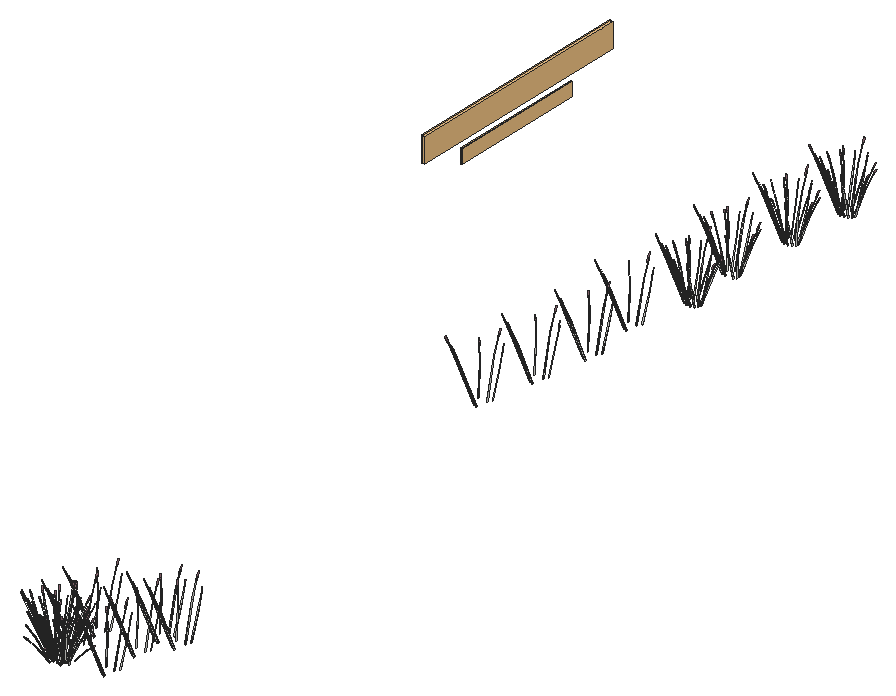
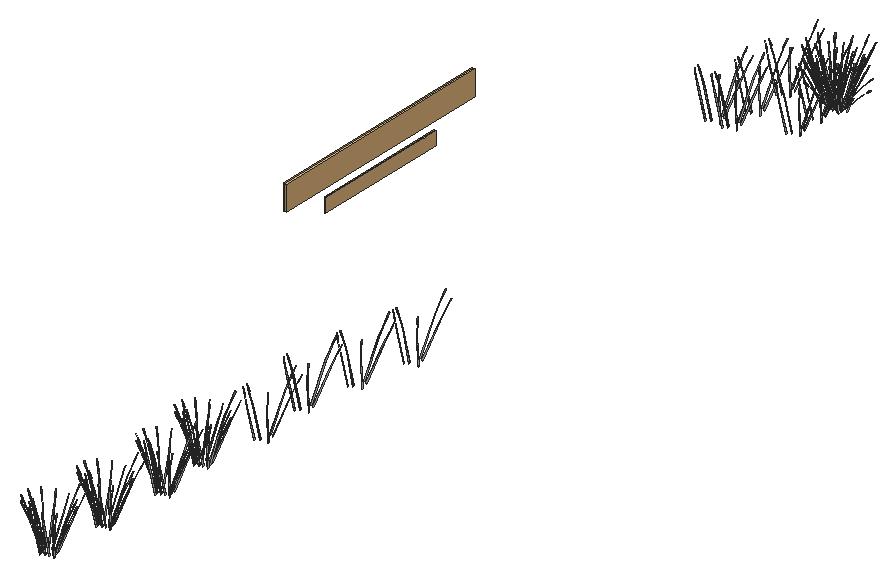
# SketchUp Ruby script. Lengths in inches.
U = 1.inch
M = Sketchup.active_model
def pt(a) = Geom::Point3d.new(a.map { |v| v * U })
def face(e, loops, mat)
  f = e.add_face(loops[0].map { |a| pt(a) })
  loops[1..].each { |l| e.add_face(l.map { |a| pt(a) }).erase! }
  f.material = f.back_material = mat if mat
  f
end
# faces: each face lists its corners as indices into pts; further lists are holes
def faces(e, pts, list, mat = nil) = list.each { |f| face(e, (f[0].is_a?(Array) ? f : [f]).map { |l| l.map { |i| pts[i] } }, mat) }
# xy, xz, yz: faces in a plane at the given z, y or x. An outline is a flat list of corners, or four numbers for a rectangle; further outlines are holes
def ring(l) = l.size == 4 ? [[l[0], l[1]], [l[2], l[1]], [l[2], l[3]], [l[0], l[3]]] : l.each_slice(2).to_a
def flat(e, list, mat, &to3) = list.each { |f| face(e, (f[0].is_a?(Array) ? f : [f]).map { |l| ring(l).map { |u, v| to3.(u, v) } }, mat) }
def xy(e, z, list, mat = nil) = flat(e, list, mat) { |x, y| [x, y, z] }
def xz(e, y, list, mat = nil) = flat(e, list, mat) { |x, z| [x, y, z] }
def yz(e, x, list, mat = nil) = flat(e, list, mat) { |y, z| [x, y, z] }
def lines(e, pts, list) = list.each { |a, b| e.add_line(pt(pts[a]), pt(pts[b])) }
# prism: a flat outline (further loops are holes) pulled along v
def prism(e, loops, v, mat = nil)
  f = face(e, loops, mat); d = Geom::Vector3d.new(v.map { |x| x * U })
  f.pushpull(f.normal.samedirection?(d) ? d.length : -d.length)
end
def box(e, o, s, mat = nil) = prism(e, [[o, [o[0] + s[0], o[1], o[2]], [o[0] + s[0], o[1] + s[1], o[2]], [o[0], o[1] + s[1], o[2]]]], [0, 0, s[2]], mat)
def at(x, y, z, deg = 0) = Geom::Transformation.translation(pt([x, y, z])) * Geom::Transformation.rotation(ORIGIN, Z_AXIS, deg.degrees)
def axes(o, x, y, z) = Geom::Transformation.new([*x, 0, *y, 0, *z, 0, *pt(o).to_a, 1])
def part(name) = M.definitions.add(name)
# library, detail: a bought-in or finely detailed component or shape, given as its bounding box
def library(name, o, s) = part(name).tap { |d| box(d.entities, o, s) }
def detail(e, o, s) = box(e.add_group.entities, o, s)
def put(e, d, t, mat = nil) = e.add_instance(d, t).tap { |i| i.material = mat if mat }
def group(e, t, mat = nil) = e.add_group.tap { |g| g.transformation = t; g.material = mat if mat }.entities
root = M.entities
M.materials.add("LightPink_Translucent").color = [144, 107, 117]
c1 = part("blade")
p = [[2.15,0.21,22],[0,0.17,0],[0.09,0.45,0],[2.18,0.31,22],[2.29,0.31,22],[0.38,0.45,0],
  [2.48,0.24,33],[2.49,0.24,33],[2.48,0.22,33]]
faces(c1.entities,p,[[0,1,2,3],[4,5,2,3],[6,3,4,7],[8,0,3,6]])
c2 = part("seeds")
p = [[0.3,-0.1,1.38],[-0.01,-0.03,1.59],[-0.01,-0.03,0.03],[0.14,-0.07,-0.07],[0.29,-0.03,3],[0.15,0.01,3.11]]
faces(c2.entities,p,[[0,1,2,3],[1,0,4,5]],"LightPink_Translucent")
c3 = part("blade with seeds")
put(c3.entities,c1,at(0,0,0))
put(c3.entities,c2,axes([2.4,0.25,30.99],[1.5799,-0.05474,1.17369],[-0.12525,1.92788,0.29478],[-0.07173,-0.02425,1.56792]))
c4 = library("WELLNESS CLUB",[0.17,0,0],[97.05,9.88,1])
c5 = library("MAXX AURA",[0.96,0,0],[68.67,9.71,1])
put(root,c3,axes([53.25,597.27,47.05],[-0.69728,-0.64842,0.35414],[0.79619,-0.61382,-0.4572],[0.40453,0.09339,0.87481]))
put(root,c3,axes([54.39,595.45,47.05],[-1.01846,-0.28891,0.35414],[0.29705,-0.84289,-0.4572],[0.41005,-0.07729,0.87481]))
put(root,c3,axes([45.72,592.11,47.05],[0.69728,0.64842,0.35414],[-0.79619,0.61382,-0.4572],[-0.40453,-0.09339,0.87481]))
put(root,c3,axes([46.18,597.63,47.05],[0.82919,-0.54528,0.35414],[0.78493,0.62262,-0.4572],[-0.11943,0.31634,0.87481]))
put(root,c3,axes([44.74,595.95,47.05],[1.06674,-0.14801,0.35414],[0.28168,0.84611,-0.4572],[-0.30569,0.22726,0.87481]))
put(root,c3,axes([51.09,598.4,47.05],[-0.18927,-0.83419,0.35414],[1.08199,-0.22027,-0.4572],[0.29062,0.23905,0.87481]))
put(root,c3,axes([54.22,593.43,47.05],[-1.06674,0.14801,0.35414],[-0.28168,-0.84611,-0.4572],[0.30569,-0.22726,0.87481]))
put(root,c3,axes([44.57,593.92,47.05],[1.01846,0.28891,0.35414],[-0.29705,0.84289,-0.4572],[-0.41005,0.07729,0.87481]))
put(root,c3,axes([52.78,591.74,47.05],[-0.82919,0.54528,0.35414],[-0.78493,-0.62262,-0.4572],[0.11943,-0.31634,0.87481]))
put(root,c3,axes([47.87,590.98,47.05],[0.18927,0.83419,0.35414],[-1.08199,0.22027,-0.4572],[-0.29062,-0.23905,0.87481]))
put(root,c3,axes([51.3,647.54,47.05],[0.36946,-0.79643,0.35414],[1.07787,0.23229,-0.4572],[0.09883,0.32066,0.87481]))
put(root,c3,axes([53.25,639.86,47.05],[-0.36946,0.79643,0.35414],[-1.07787,-0.23229,-0.4572],[-0.09883,-0.32066,0.87481]))
put(root,c3,axes([56.04,646.28,47.05],[-0.69728,-0.64842,0.35414],[0.79619,-0.61382,-0.4572],[0.40453,0.09339,0.87481]))
put(root,c3,axes([57.1875,644.46,47.05],[-1.01846,-0.28891,0.35414],[0.29705,-0.84289,-0.4572],[0.41005,-0.07729,0.87481]))
put(root,c3,axes([48.51,641.12,47.05],[0.69728,0.64842,0.35414],[-0.79619,0.61382,-0.4572],[-0.40453,-0.09339,0.87481]))
put(root,c3,axes([48.97,646.64,47.05],[0.82919,-0.54528,0.35414],[0.78493,0.62262,-0.4572],[-0.11943,0.31634,0.87481]))
put(root,c3,axes([47.53,644.96,47.05],[1.06674,-0.14801,0.35414],[0.28168,0.84611,-0.4572],[-0.30569,0.22726,0.87481]))
put(root,c3,axes([53.88,647.41,47.05],[-0.18927,-0.83419,0.35414],[1.08199,-0.22027,-0.4572],[0.29062,0.23905,0.87481]))
put(root,c3,axes([57.02,642.44,47.05],[-1.06674,0.14801,0.35414],[-0.28168,-0.84611,-0.4572],[0.30569,-0.22726,0.87481]))
put(root,c3,axes([47.36,642.93,47.05],[1.01846,0.28891,0.35414],[-0.29705,0.84289,-0.4572],[-0.41005,0.07729,0.87481]))
put(root,c3,axes([55.58,640.75,47.05],[-0.82919,0.54528,0.35414],[-0.78493,-0.62262,-0.4572],[0.11943,-0.31634,0.87481]))
put(root,c3,axes([50.66,639.99,47.05],[0.18927,0.83419,0.35414],[-1.08199,0.22027,-0.4572],[-0.29062,-0.23905,0.87481]))
put(root,c3,axes([55.84,691.87,47.05],[0.36946,-0.79643,0.35414],[1.07787,0.23229,-0.4572],[0.09883,0.32066,0.87481]))
put(root,c3,axes([57.79,684.1875,47.05],[-0.36946,0.79643,0.35414],[-1.07787,-0.23229,-0.4572],[-0.09883,-0.32066,0.87481]))
put(root,c3,axes([60.58,690.61,47.05],[-0.69728,-0.64842,0.35414],[0.79619,-0.61382,-0.4572],[0.40453,0.09339,0.87481]))
put(root,c3,axes([61.73,688.79,47.05],[-1.01846,-0.28891,0.35414],[0.29705,-0.84289,-0.4572],[0.41005,-0.07729,0.87481]))
put(root,c3,axes([53.05,685.44,47.05],[0.69728,0.64842,0.35414],[-0.79619,0.61382,-0.4572],[-0.40453,-0.09339,0.87481]))
put(root,c3,axes([53.51,690.97,47.05],[0.82919,-0.54528,0.35414],[0.78493,0.62262,-0.4572],[-0.11943,0.31634,0.87481]))
put(root,c3,axes([52.07,689.29,47.05],[1.06674,-0.14801,0.35414],[0.28168,0.84611,-0.4572],[-0.30569,0.22726,0.87481]))
put(root,c3,axes([58.42,691.74,47.05],[-0.18927,-0.83419,0.35414],[1.08199,-0.22027,-0.4572],[0.29062,0.23905,0.87481]))
put(root,c3,axes([61.56,686.77,47.05],[-1.06674,0.14801,0.35414],[-0.28168,-0.84611,-0.4572],[0.30569,-0.22726,0.87481]))
put(root,c3,axes([51.9,687.26,47.05],[1.01846,0.28891,0.35414],[-0.29705,0.84289,-0.4572],[-0.41005,0.07729,0.87481]))
put(root,c3,axes([60.12,685.08,47.05],[-0.82919,0.54528,0.35414],[-0.78493,-0.62262,-0.4572],[0.11943,-0.31634,0.87481]))
put(root,c3,axes([55.2,684.32,47.05],[0.18927,0.83419,0.35414],[-1.08199,0.22027,-0.4572],[-0.29062,-0.23905,0.87481]))
put(root,c3,axes([52.33,559.71,47.05],[0.36946,-0.79643,0.35414],[1.07787,0.23229,-0.4572],[0.09883,0.32066,0.87481]))
put(root,c3,axes([54.29,552.02,47.05],[-0.36946,0.79643,0.35414],[-1.07787,-0.23229,-0.4572],[-0.09883,-0.32066,0.87481]))
put(root,c3,axes([57.08,558.45,47.05],[-0.69728,-0.64842,0.35414],[0.79619,-0.61382,-0.4572],[0.40453,0.09339,0.87481]))
put(root,c3,axes([58.22,556.63,47.05],[-1.01846,-0.28891,0.35414],[0.29705,-0.84289,-0.4572],[0.41005,-0.07729,0.87481]))
put(root,c3,axes([49.55,553.28,47.05],[0.69728,0.64842,0.35414],[-0.79619,0.61382,-0.4572],[-0.40453,-0.09339,0.87481]))
put(root,c3,axes([50.01,558.81,47.05],[0.82919,-0.54528,0.35414],[0.78493,0.62262,-0.4572],[-0.11943,0.31634,0.87481]))
put(root,c3,axes([48.57,557.12,47.05],[1.06674,-0.14801,0.35414],[0.28168,0.84611,-0.4572],[-0.30569,0.22726,0.87481]))
put(root,c3,axes([54.92,559.57,47.05],[-0.18927,-0.83419,0.35414],[1.08199,-0.22027,-0.4572],[0.29062,0.23905,0.87481]))
put(root,c3,axes([58.05,554.6,47.05],[-1.06674,0.14801,0.35414],[-0.28168,-0.84611,-0.4572],[0.30569,-0.22726,0.87481]))
put(root,c3,axes([48.4,555.1,47.05],[1.01846,0.28891,0.35414],[-0.29705,0.84289,-0.4572],[-0.41005,0.07729,0.87481]))
put(root,c3,axes([56.61,552.92,47.05],[-0.82919,0.54528,0.35414],[-0.78493,-0.62262,-0.4572],[0.11943,-0.31634,0.87481]))
put(root,c3,axes([51.7,552.15,47.05],[0.18927,0.83419,0.35414],[-1.08199,0.22027,-0.4572],[-0.29062,-0.23905,0.87481]))
put(root,c3,axes([24.8,17.97,46.96],[0.09085,0.10335,1.77383],[-0.43798,0.92907,-0.16761],[-0.44357,0.00672,0.31391]))
put(root,c3,axes([28.63,15.28,46.96],[-0.02286,0.12414,1.77383],[-1.12758,0.45052,-0.16761],[-0.33182,-0.23029,0.31391]))
put(root,c3,axes([31.04,27.05,46.96],[0.00363,-0.12539,1.77383],[1.0502,-0.55319,-0.16761],[0.36479,0.19745,0.31391]))
put(root,c3,axes([21.63,23.06,46.96],[0.1564,0.02778,1.77383],[0.48382,0.91506,-0.16761],[-0.32016,0.24017,0.31391]))
put(root,c3,axes([38.57,20.74,46.96],[-0.16006,-0.00787,1.77383],[-0.66468,-0.8428,-0.16761],[0.26693,-0.27711,0.31391]))
put(root,c3,axes([38.28,26.01,46.96],[-0.11081,-0.09067,1.77383],[0.2424,-0.97188,-0.16761],[0.43649,-0.06209,0.31391]))
put(root,c3,axes([23.79,27.83,46.96],[0.13903,-0.06253,1.77383],[1.14912,0.41591,-0.16761],[-0.027,0.34629,0.31391]))
put(root,c3,axes([35.27,16.8,46.96],[-0.12446,0.07911,1.77383],[-1.21937,-0.26689,-0.16761],[-0.04414,-0.34521,0.31391]))
put(root,c3,axes([26.65,25.27,47.65],[1.34686,0.05131,-0.13498],[-0.03681,0.97156,-0.74919],[-0.09356,0.37418,1.13838]))
put(root,c3,axes([28.95,17.64,47.68],[-0.81789,0.99285,-0.13619],[-1.18445,-0.572,-0.75594],[-0.41173,-0.28051,1.14864]))
put(root,c3,axes([28.7,17.71,46.98],[0.55698,-0.6579,0.0643],[0.79316,0.38303,0.50621],[-0.25643,-0.21093,0.77189]))
put(root,c3,axes([29.17,26.74,46.98],[-0.90301,0.35198,0.0643],[-0.44199,-0.64184,0.50621],[0.08721,0.28293,0.77189]))
put(root,c3,axes([36.19,20.78,46.98],[0.8413,0.43556,0.0643],[-0.48981,0.62025,0.50621],[0.26973,-0.20053,0.77189]))
put(root,c3,axes([36.32,23.2,46.98],[0.4501,0.70615,0.0643],[-0.82077,0.34564,0.50621],[0.36181,-0.0682,0.77189]))
put(root,c3,axes([26.08,19,46.98],[0.06171,-0.78753,0.0643],[0.9318,0.02159,0.50621],[-0.35694,-0.08241,0.77189]))
put(root,c3,axes([34.54,18.73,46.98],[1.00708,0.04826,0.0643],[-0.02761,0.72867,0.50621],[0.10538,-0.27912,0.77189]))
put(root,c3,axes([34.88,25.34,46.98],[-0.06171,0.78753,0.0643],[-0.9318,-0.02159,0.50621],[0.35694,0.08241,0.77189]))
put(root,c3,axes([24.77,23.57,46.98],[-0.8413,-0.43556,0.0643],[0.48981,-0.62025,0.50621],[-0.26973,0.20053,0.77189]))
put(root,c3,axes([31.79,17.61,46.98],[0.90301,-0.35198,0.0643],[0.44199,0.64184,0.50621],[-0.08721,-0.28293,0.77189]))
put(root,c3,axes([24.65,21.15,46.98],[-0.4501,-0.70615,0.0643],[0.82077,-0.34564,0.50621],[-0.36181,0.0682,0.77189]))
put(root,c3,axes([32.26,26.64,46.98],[-0.55698,0.6579,0.0643],[-0.79316,-0.38303,0.50621],[0.25643,0.21093,0.77189]))
put(root,c3,axes([26.43,25.61,46.98],[-1.00708,-0.04826,0.0643],[0.02761,-0.72867,0.50621],[-0.10538,0.27912,0.77189]))
put(root,c3,axes([31.47,17.68,46.98],[1.20755,0.27075,0.48003],[-0.41292,0.89013,0.3958],[-0.07257,-0.35005,0.9933]))
put(root,c3,axes([34.97,25.09,46.98],[-0.90362,0.68241,0.48003],[-0.77932,-0.72471,0.3958],[0.42395,0.12588,0.9933]))
put(root,c3,axes([36.23,22.95,46.98],[-0.34623,0.9443,0.48003],[-1.13828,-0.3229,0.3958],[0.44763,-0.05675,0.9933]))
put(root,c3,axes([25.01,23.75,46.98],[-0.30393,-0.95317,0.48003],[1.19224,-0.16542,0.3958],[-0.35138,0.22417,0.9933]))
put(root,c3,axes([26.75,25.68,46.98],[-0.87265,-0.70663,0.48003],[0.92674,-0.60943,0.3958],[-0.16097,0.33153,0.9933]))
put(root,c3,axes([34.22,18.67,46.98],[0.87265,0.70663,0.48003],[-0.92674,0.60943,0.3958],[0.16097,-0.33153,0.9933]))
put(root,c3,axes([24.73,21.4,46.98],[0.34623,-0.9443,0.48003],[1.13828,0.3229,0.3958],[-0.44763,0.05675,0.9933]))
put(root,c3,axes([35.96,20.6,46.98],[0.30393,0.95317,0.48003],[-1.19224,0.16542,0.3958],[0.35138,-0.22417,0.9933]))
put(root,c3,axes([32.5,26.45,46.98],[-1.21888,0.23767,0.48003],[-0.21154,-0.93233,0.3958],[0.28666,0.27478,0.9933]))
put(root,c3,axes([31.04,42.73,47.0625],[-1.20755,-0.27075,0.53283],[0.41292,-0.89013,0.43934],[0.07257,0.35005,1.10256]))
put(root,c3,axes([30.74,61.76,47.0625],[-1.20755,-0.27075,0.53283],[0.41292,-0.89013,0.43934],[0.07257,0.35005,1.10256]))
put(root,c3,axes([62.51,30.73,47.0625],[-1.20755,-0.27075,0.53283],[0.41292,-0.89013,0.43934],[0.07257,0.35005,1.10256]))
put(root,c3,axes([62.3,58.02,47.0625],[-1.20755,-0.27075,0.53283],[0.41292,-0.89013,0.43934],[0.07257,0.35005,1.10256]))
put(root,c3,axes([62.3,78.73,47.0625],[-1.20755,-0.27075,0.53283],[0.41292,-0.89013,0.43934],[0.07257,0.35005,1.10256]))
put(root,c3,axes([74.3,78.73,47.0625],[-1.20755,-0.27075,0.53283],[0.41292,-0.89013,0.43934],[0.07257,0.35005,1.10256]))
put(root,c3,axes([33.46,397.47,47.0625],[-1.20755,-0.27075,0.53283],[0.41292,-0.89013,0.43934],[0.07257,0.35005,1.10256]))
put(root,c3,axes([41.61,437.16,47.0625],[-1.20755,-0.27075,0.53283],[0.41292,-0.89013,0.43934],[0.07257,0.35005,1.10256]))
put(root,c3,axes([47.97,476.43,47.0625],[-1.20755,-0.27075,0.53283],[0.41292,-0.89013,0.43934],[0.07257,0.35005,1.10256]))
put(root,c3,axes([44.35,516.68,47.0625],[-1.20755,-0.27075,0.53283],[0.41292,-0.89013,0.43934],[0.07257,0.35005,1.10256]))
put(root,c3,axes([48.49,599.18,47.0625],[-1.20755,-0.27075,0.53283],[0.41292,-0.89013,0.43934],[0.07257,0.35005,1.10256]))
put(root,c3,axes([51.28,648.19,47.0625],[-1.20755,-0.27075,0.53283],[0.41292,-0.89013,0.43934],[0.07257,0.35005,1.10256]))
put(root,c3,axes([55.82,692.52,47.0625],[-1.20755,-0.27075,0.53283],[0.41292,-0.89013,0.43934],[0.07257,0.35005,1.10256]))
put(root,c3,axes([52.32,560.36,47.0625],[-1.20755,-0.27075,0.53283],[0.41292,-0.89013,0.43934],[0.07257,0.35005,1.10256]))
put(root,c3,axes([27.17,35.07,47.09],[1.01205,-0.7643,0.53763],[0.87284,0.81167,0.4433],[-0.47482,-0.14098,1.11249]))
put(root,c3,axes([29.93,33.54,47.09],[1.36515,-0.26619,0.53763],[0.23692,1.04421,0.4433],[-0.32106,-0.30775,1.11249]))
put(root,c3,axes([26.87,54.1,47.09],[1.01205,-0.7643,0.53763],[0.87284,0.81167,0.4433],[-0.47482,-0.14098,1.11249]))
put(root,c3,axes([29.63,52.57,47.09],[1.36515,-0.26619,0.53763],[0.23692,1.04421,0.4433],[-0.32106,-0.30775,1.11249]))
put(root,c3,axes([58.64,23.07,47.09],[1.01205,-0.7643,0.53763],[0.87284,0.81167,0.4433],[-0.47482,-0.14098,1.11249]))
put(root,c3,axes([61.4,21.54,47.09],[1.36515,-0.26619,0.53763],[0.23692,1.04421,0.4433],[-0.32106,-0.30775,1.11249]))
put(root,c3,axes([58.43,50.35,47.09],[1.01205,-0.7643,0.53763],[0.87284,0.81167,0.4433],[-0.47482,-0.14098,1.11249]))
put(root,c3,axes([61.2,48.83,47.09],[1.36515,-0.26619,0.53763],[0.23692,1.04421,0.4433],[-0.32106,-0.30775,1.11249]))
put(root,c3,axes([58.43,71.07,47.09],[1.01205,-0.7643,0.53763],[0.87284,0.81167,0.4433],[-0.47482,-0.14098,1.11249]))
put(root,c3,axes([61.2,69.54,47.09],[1.36515,-0.26619,0.53763],[0.23692,1.04421,0.4433],[-0.32106,-0.30775,1.11249]))
put(root,c3,axes([70.43,71.07,47.09],[1.01205,-0.7643,0.53763],[0.87284,0.81167,0.4433],[-0.47482,-0.14098,1.11249]))
put(root,c3,axes([73.2,69.54,47.09],[1.36515,-0.26619,0.53763],[0.23692,1.04421,0.4433],[-0.32106,-0.30775,1.11249]))
put(root,c3,axes([29.59,389.81,47.09],[1.01205,-0.7643,0.53763],[0.87284,0.81167,0.4433],[-0.47482,-0.14098,1.11249]))
put(root,c3,axes([32.35,388.28,47.09],[1.36515,-0.26619,0.53763],[0.23692,1.04421,0.4433],[-0.32106,-0.30775,1.11249]))
put(root,c3,axes([37.74,429.5,47.09],[1.01205,-0.7643,0.53763],[0.87284,0.81167,0.4433],[-0.47482,-0.14098,1.11249]))
put(root,c3,axes([40.51,427.97,47.09],[1.36515,-0.26619,0.53763],[0.23692,1.04421,0.4433],[-0.32106,-0.30775,1.11249]))
put(root,c3,axes([44.1,468.76,47.09],[1.01205,-0.7643,0.53763],[0.87284,0.81167,0.4433],[-0.47482,-0.14098,1.11249]))
put(root,c3,axes([46.86,467.24,47.09],[1.36515,-0.26619,0.53763],[0.23692,1.04421,0.4433],[-0.32106,-0.30775,1.11249]))
put(root,c3,axes([40.48,509.02,47.09],[1.01205,-0.7643,0.53763],[0.87284,0.81167,0.4433],[-0.47482,-0.14098,1.11249]))
put(root,c3,axes([43.25,507.5,47.09],[1.36515,-0.26619,0.53763],[0.23692,1.04421,0.4433],[-0.32106,-0.30775,1.11249]))
put(root,c3,axes([44.62,591.52,47.09],[1.01205,-0.7643,0.53763],[0.87284,0.81167,0.4433],[-0.47482,-0.14098,1.11249]))
put(root,c3,axes([47.39,590,47.09],[1.36515,-0.26619,0.53763],[0.23692,1.04421,0.4433],[-0.32106,-0.30775,1.11249]))
put(root,c3,axes([47.41,640.53,47.09],[1.01205,-0.7643,0.53763],[0.87284,0.81167,0.4433],[-0.47482,-0.14098,1.11249]))
put(root,c3,axes([50.18,639.01,47.09],[1.36515,-0.26619,0.53763],[0.23692,1.04421,0.4433],[-0.32106,-0.30775,1.11249]))
put(root,c3,axes([51.95,684.86,47.09],[1.01205,-0.7643,0.53763],[0.87284,0.81167,0.4433],[-0.47482,-0.14098,1.11249]))
put(root,c3,axes([54.72,683.34,47.09],[1.36515,-0.26619,0.53763],[0.23692,1.04421,0.4433],[-0.32106,-0.30775,1.11249]))
put(root,c3,axes([48.45,552.7,47.09],[1.01205,-0.7643,0.53763],[0.87284,0.81167,0.4433],[-0.47482,-0.14098,1.11249]))
put(root,c3,axes([51.22,551.17,47.09],[1.36515,-0.26619,0.53763],[0.23692,1.04421,0.4433],[-0.32106,-0.30775,1.11249]))
put(root,c3,axes([29.5,26.02,47.3],[0.36946,-0.79643,0.35414],[1.07787,0.23229,-0.4572],[0.09883,0.32066,0.87481]))
put(root,c3,axes([31.46,18.33,47.3],[-0.36946,0.79643,0.35414],[-1.07787,-0.23229,-0.4572],[-0.09883,-0.32066,0.87481]))
put(root,c3,axes([34.25,24.76,47.3],[-0.69728,-0.64842,0.35414],[0.79619,-0.61382,-0.4572],[0.40453,0.09339,0.87481]))
put(root,c3,axes([35.39,22.9375,47.3],[-1.01846,-0.28891,0.35414],[0.29705,-0.84289,-0.4572],[0.41005,-0.07729,0.87481]))
put(root,c3,axes([26.72,19.59,47.3],[0.69728,0.64842,0.35414],[-0.79619,0.61382,-0.4572],[-0.40453,-0.09339,0.87481]))
put(root,c3,axes([27.18,25.12,47.3],[0.82919,-0.54528,0.35414],[0.78493,0.62262,-0.4572],[-0.11943,0.31634,0.87481]))
put(root,c3,axes([25.74,23.43,47.3],[1.06674,-0.14801,0.35414],[0.28168,0.84611,-0.4572],[-0.30569,0.22726,0.87481]))
put(root,c3,axes([32.09,25.88,47.3],[-0.18927,-0.83419,0.35414],[1.08199,-0.22027,-0.4572],[0.29062,0.23905,0.87481]))
put(root,c3,axes([35.23,20.91,47.3],[-1.06674,0.14801,0.35414],[-0.28168,-0.84611,-0.4572],[0.30569,-0.22726,0.87481]))
put(root,c3,axes([25.57,21.41,47.3],[1.01846,0.28891,0.35414],[-0.29705,0.84289,-0.4572],[-0.41005,0.07729,0.87481]))
put(root,c3,axes([33.78,19.23,47.3],[-0.82919,0.54528,0.35414],[-0.78493,-0.62262,-0.4572],[0.11943,-0.31634,0.87481]))
put(root,c3,axes([28.87,18.46,47.3],[0.18927,0.83419,0.35414],[-1.08199,0.22027,-0.4572],[-0.29062,-0.23905,0.87481]))
put(root,c3,axes([29.49,26.67,47.3125],[-1.20755,-0.27075,0.53283],[0.41292,-0.89013,0.43934],[0.07257,0.35005,1.10256]))
put(root,c3,axes([32.5,44.92,47.65],[0.84686,-0.59414,-0.06488],[0.77596,0.65071,-0.29416],[0.05463,0.18438,0.97024]))
put(root,c3,axes([24.86,41.9,47.65],[1.08141,0.27645,-0.06488],[-0.33265,0.85086,-0.29416],[-0.17688,0.12919,0.97024]))
put(root,c3,axes([32.2,63.95,47.65],[0.84686,-0.59414,-0.06488],[0.77596,0.65071,-0.29416],[0.05463,0.18438,0.97024]))
put(root,c3,axes([24.5625,60.93,47.65],[1.08141,0.27645,-0.06488],[-0.33265,0.85086,-0.29416],[-0.17688,0.12919,0.97024]))
put(root,c3,axes([63.97,32.92,47.65],[0.84686,-0.59414,-0.06488],[0.77596,0.65071,-0.29416],[0.05463,0.18438,0.97024]))
put(root,c3,axes([56.33,29.9,47.65],[1.08141,0.27645,-0.06488],[-0.33265,0.85086,-0.29416],[-0.17688,0.12919,0.97024]))
put(root,c3,axes([63.76,60.2,47.65],[0.84686,-0.59414,-0.06488],[0.77596,0.65071,-0.29416],[0.05463,0.18438,0.97024]))
put(root,c3,axes([56.125,57.18,47.65],[1.08141,0.27645,-0.06488],[-0.33265,0.85086,-0.29416],[-0.17688,0.12919,0.97024]))
put(root,c3,axes([63.76,80.92,47.65],[0.84686,-0.59414,-0.06488],[0.77596,0.65071,-0.29416],[0.05463,0.18438,0.97024]))
put(root,c3,axes([56.125,77.9,47.65],[1.08141,0.27645,-0.06488],[-0.33265,0.85086,-0.29416],[-0.17688,0.12919,0.97024]))
put(root,c3,axes([75.76,80.92,47.65],[0.84686,-0.59414,-0.06488],[0.77596,0.65071,-0.29416],[0.05463,0.18438,0.97024]))
put(root,c3,axes([68.125,77.9,47.65],[1.08141,0.27645,-0.06488],[-0.33265,0.85086,-0.29416],[-0.17688,0.12919,0.97024]))
put(root,c3,axes([34.92,399.66,47.65],[0.84686,-0.59414,-0.06488],[0.77596,0.65071,-0.29416],[0.05463,0.18438,0.97024]))
put(root,c3,axes([27.29,396.63,47.65],[1.08141,0.27645,-0.06488],[-0.33265,0.85086,-0.29416],[-0.17688,0.12919,0.97024]))
put(root,c3,axes([43.08,439.35,47.65],[0.84686,-0.59414,-0.06488],[0.77596,0.65071,-0.29416],[0.05463,0.18438,0.97024]))
put(root,c3,axes([35.4375,436.33,47.65],[1.08141,0.27645,-0.06488],[-0.33265,0.85086,-0.29416],[-0.17688,0.12919,0.97024]))
put(root,c3,axes([49.43,478.61,47.65],[0.84686,-0.59414,-0.06488],[0.77596,0.65071,-0.29416],[0.05463,0.18438,0.97024]))
put(root,c3,axes([41.79,475.59,47.65],[1.08141,0.27645,-0.06488],[-0.33265,0.85086,-0.29416],[-0.17688,0.12919,0.97024]))
put(root,c3,axes([45.82,518.87,47.65],[0.84686,-0.59414,-0.06488],[0.77596,0.65071,-0.29416],[0.05463,0.18438,0.97024]))
put(root,c3,axes([38.18,515.85,47.65],[1.08141,0.27645,-0.06488],[-0.33265,0.85086,-0.29416],[-0.17688,0.12919,0.97024]))
put(root,c3,axes([49.95,601.37,47.65],[0.84686,-0.59414,-0.06488],[0.77596,0.65071,-0.29416],[0.05463,0.18438,0.97024]))
put(root,c3,axes([42.32,598.35,47.65],[1.08141,0.27645,-0.06488],[-0.33265,0.85086,-0.29416],[-0.17688,0.12919,0.97024]))
put(root,c3,axes([52.75,650.38,47.65],[0.84686,-0.59414,-0.06488],[0.77596,0.65071,-0.29416],[0.05463,0.18438,0.97024]))
put(root,c3,axes([45.11,647.36,47.65],[1.08141,0.27645,-0.06488],[-0.33265,0.85086,-0.29416],[-0.17688,0.12919,0.97024]))
put(root,c3,axes([57.29,694.71,47.65],[0.84686,-0.59414,-0.06488],[0.77596,0.65071,-0.29416],[0.05463,0.18438,0.97024]))
put(root,c3,axes([49.65,691.6875,47.65],[1.08141,0.27645,-0.06488],[-0.33265,0.85086,-0.29416],[-0.17688,0.12919,0.97024]))
put(root,c3,axes([53.78,562.55,47.65],[0.84686,-0.59414,-0.06488],[0.77596,0.65071,-0.29416],[0.05463,0.18438,0.97024]))
put(root,c3,axes([46.15,559.52,47.65],[1.08141,0.27645,-0.06488],[-0.33265,0.85086,-0.29416],[-0.17688,0.12919,0.97024]))
put(root,c3,axes([25.625,19.01,47.34],[1.01205,-0.7643,0.53763],[0.87284,0.81167,0.4433],[-0.47482,-0.14098,1.11249]))
put(root,c3,axes([28.39,17.48,47.34],[1.36515,-0.26619,0.53763],[0.23692,1.04421,0.4433],[-0.32106,-0.30775,1.11249]))
put(root,c3,axes([30.95,28.86,47.9],[0.84686,-0.59414,-0.06488],[0.77596,0.65071,-0.29416],[0.05463,0.18438,0.97024]))
put(root,c3,axes([23.32,25.84,47.9],[1.08141,0.27645,-0.06488],[-0.33265,0.85086,-0.29416],[-0.17688,0.12919,0.97024]))
put(root,c4,axes([14.89,397.1,192.14],[0,1,0],[0,0,1],[1,0,0]))
put(root,c5,axes([14.89,359.86,208.11],[0,2.4271,0],[0,0,1.78723],[2.20646,0,0]))
